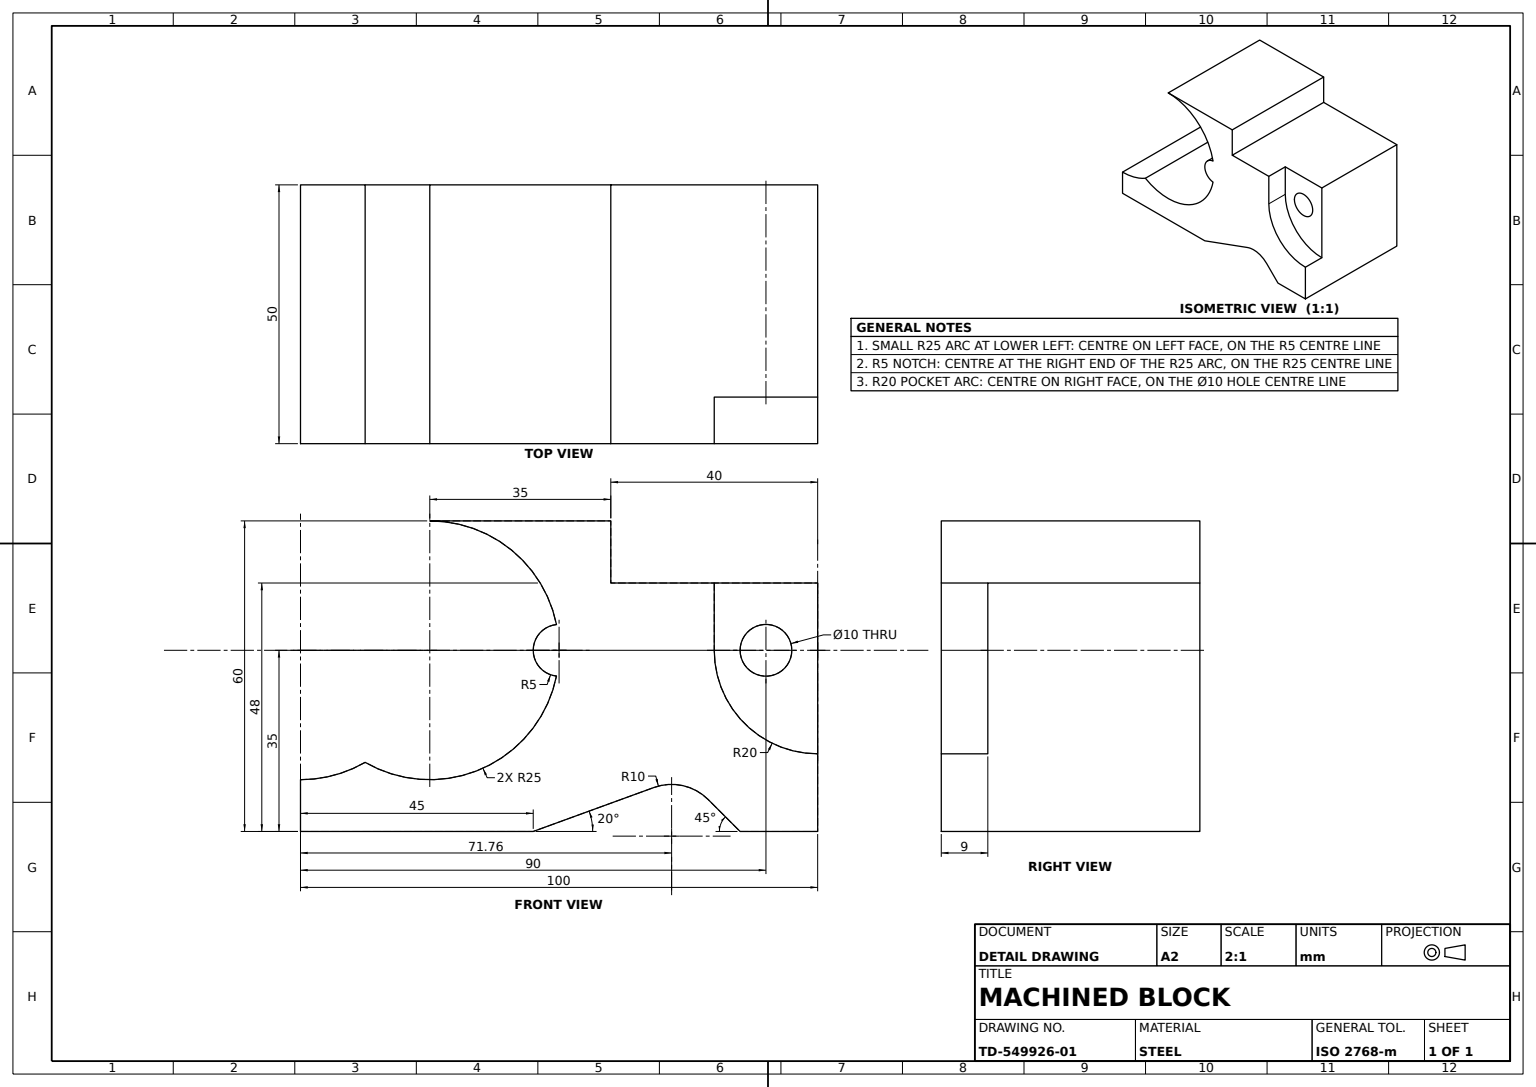
ISO-10303-21;
HEADER;
FILE_DESCRIPTION((''),'2;1');
FILE_NAME('','',(''),(''),'','','');
FILE_SCHEMA(('AUTOMOTIVE_DESIGN'));
ENDSEC;
DATA;
#1=APPLICATION_CONTEXT('');
#2=PRODUCT_CONTEXT('',#1,'mechanical');
#3=PRODUCT('','','',(#2));
#4=PRODUCT_DEFINITION_FORMATION('','',#3);
#5=PRODUCT_DEFINITION_CONTEXT('',#1,'design');
#6=PRODUCT_DEFINITION('','',#4,#5);
#7=PRODUCT_DEFINITION_SHAPE('','',#6);
#8=(LENGTH_UNIT()NAMED_UNIT(*)SI_UNIT(.MILLI.,.METRE.));
#9=(NAMED_UNIT(*)PLANE_ANGLE_UNIT()SI_UNIT($,.RADIAN.));
#10=(NAMED_UNIT(*)SI_UNIT($,.STERADIAN.)SOLID_ANGLE_UNIT());
#11=UNCERTAINTY_MEASURE_WITH_UNIT(LENGTH_MEASURE(1.E-05),#8,'distance_accuracy_value','');
#12=(GEOMETRIC_REPRESENTATION_CONTEXT(3)GLOBAL_UNCERTAINTY_ASSIGNED_CONTEXT((#11))GLOBAL_UNIT_ASSIGNED_CONTEXT((#8,#9,#10))REPRESENTATION_CONTEXT('',''));
#13=CARTESIAN_POINT('',(85.,35.,-25.));
#14=VERTEX_POINT('',#13);
#15=CARTESIAN_POINT('',(85.,35.,16.));
#16=VERTEX_POINT('',#15);
#17=CARTESIAN_POINT('',(85.,35.,-101.));
#18=DIRECTION('',(0.,0.,1.));
#19=VECTOR('',#18,1000.);
#20=LINE('',#17,#19);
#21=EDGE_CURVE('',#14,#16,#20,.T.);
#22=ORIENTED_EDGE('',*,*,#21,.F.);
#23=CARTESIAN_POINT('',(95.,35.,-25.));
#24=VERTEX_POINT('',#23);
#25=CARTESIAN_POINT('',(90.,35.,-25.));
#26=DIRECTION('',(1.,0.,0.));
#27=AXIS2_PLACEMENT_3D('',#25,#18,#26);
#28=CIRCLE('',#27,5.);
#29=EDGE_CURVE('',#24,#14,#28,.T.);
#30=ORIENTED_EDGE('',*,*,#29,.F.);
#31=CARTESIAN_POINT('',(95.,35.,16.));
#32=VERTEX_POINT('',#31);
#33=CARTESIAN_POINT('',(95.,35.,-101.));
#34=LINE('',#33,#19);
#35=EDGE_CURVE('',#24,#32,#34,.T.);
#36=ORIENTED_EDGE('',*,*,#35,.T.);
#37=CARTESIAN_POINT('',(90.,35.,16.));
#38=AXIS2_PLACEMENT_3D('',#37,#18,#26);
#39=CIRCLE('',#38,5.);
#40=EDGE_CURVE('',#32,#16,#39,.T.);
#41=ORIENTED_EDGE('',*,*,#40,.T.);
#42=EDGE_LOOP('',(#22,#30,#36,#41));
#43=FACE_OUTER_BOUND('',#42,.T.);
#44=CARTESIAN_POINT('',(90.,35.,-101.));
#45=AXIS2_PLACEMENT_3D('',#44,#18,#26);
#46=CYLINDRICAL_SURFACE('',#45,5.);
#47=ADVANCED_FACE('',(#43),#46,.F.);
#48=CARTESIAN_POINT('',(0.,0.,25.));
#49=VERTEX_POINT('',#48);
#50=CARTESIAN_POINT('',(0.,0.,-25.));
#51=VERTEX_POINT('',#50);
#52=DIRECTION('',(0.,0.,-1.));
#53=VECTOR('',#52,1000.);
#54=LINE('',#48,#53);
#55=EDGE_CURVE('',#49,#51,#54,.T.);
#56=ORIENTED_EDGE('',*,*,#55,.T.);
#57=CARTESIAN_POINT('',(45.,0.,-25.));
#58=VERTEX_POINT('',#57);
#59=VECTOR('',#26,1000.);
#60=LINE('',#50,#59);
#61=EDGE_CURVE('',#51,#58,#60,.T.);
#62=ORIENTED_EDGE('',*,*,#61,.T.);
#63=CARTESIAN_POINT('',(45.,0.,25.));
#64=VERTEX_POINT('',#63);
#65=LINE('',#57,#19);
#66=EDGE_CURVE('',#58,#64,#65,.T.);
#67=ORIENTED_EDGE('',*,*,#66,.T.);
#68=LINE('',#48,#59);
#69=EDGE_CURVE('',#49,#64,#68,.T.);
#70=ORIENTED_EDGE('',*,*,#69,.F.);
#71=EDGE_LOOP('',(#56,#62,#67,#70));
#72=FACE_OUTER_BOUND('',#71,.T.);
#73=DIRECTION('',(0.,1.,0.));
#74=AXIS2_PLACEMENT_3D('',#48,#73,#18);
#75=PLANE('',#74);
#76=ADVANCED_FACE('',(#72),#75,.F.);
#77=CARTESIAN_POINT('',(25.,60.,25.));
#78=VERTEX_POINT('',#77);
#79=CARTESIAN_POINT('',(25.,60.,-25.));
#80=VERTEX_POINT('',#79);
#81=LINE('',#77,#53);
#82=EDGE_CURVE('',#78,#80,#81,.T.);
#83=ORIENTED_EDGE('',*,*,#82,.F.);
#84=CARTESIAN_POINT('',(60.,60.,25.));
#85=VERTEX_POINT('',#84);
#86=CARTESIAN_POINT('',(0.,60.,25.));
#87=LINE('',#86,#59);
#88=EDGE_CURVE('',#78,#85,#87,.T.);
#89=ORIENTED_EDGE('',*,*,#88,.T.);
#90=CARTESIAN_POINT('',(60.,60.,-25.));
#91=VERTEX_POINT('',#90);
#92=LINE('',#84,#53);
#93=EDGE_CURVE('',#85,#91,#92,.T.);
#94=ORIENTED_EDGE('',*,*,#93,.T.);
#95=CARTESIAN_POINT('',(0.,60.,-25.));
#96=LINE('',#95,#59);
#97=EDGE_CURVE('',#80,#91,#96,.T.);
#98=ORIENTED_EDGE('',*,*,#97,.F.);
#99=EDGE_LOOP('',(#83,#89,#94,#98));
#100=FACE_OUTER_BOUND('',#99,.T.);
#101=AXIS2_PLACEMENT_3D('',#86,#73,#18);
#102=PLANE('',#101);
#103=ADVANCED_FACE('',(#100),#102,.T.);
#104=CARTESIAN_POINT('',(0.,10.,25.));
#105=VERTEX_POINT('',#104);
#106=CARTESIAN_POINT('',(0.,10.,-25.));
#107=VERTEX_POINT('',#106);
#108=LINE('',#104,#53);
#109=EDGE_CURVE('',#105,#107,#108,.T.);
#110=ORIENTED_EDGE('',*,*,#109,.F.);
#111=CARTESIAN_POINT('',(12.5,13.349365,25.));
#112=VERTEX_POINT('',#111);
#113=CARTESIAN_POINT('',(0.,35.,25.));
#114=AXIS2_PLACEMENT_3D('',#113,#18,#26);
#115=CIRCLE('',#114,25.);
#116=EDGE_CURVE('',#105,#112,#115,.T.);
#117=ORIENTED_EDGE('',*,*,#116,.T.);
#118=CARTESIAN_POINT('',(12.5,13.349365,-25.));
#119=VERTEX_POINT('',#118);
#120=CARTESIAN_POINT('',(12.5,13.349365,0.));
#121=LINE('',#120,#19);
#122=EDGE_CURVE('',#119,#112,#121,.T.);
#123=ORIENTED_EDGE('',*,*,#122,.F.);
#124=CARTESIAN_POINT('',(0.,35.,-25.));
#125=AXIS2_PLACEMENT_3D('',#124,#18,#26);
#126=CIRCLE('',#125,25.);
#127=EDGE_CURVE('',#107,#119,#126,.T.);
#128=ORIENTED_EDGE('',*,*,#127,.F.);
#129=EDGE_LOOP('',(#110,#117,#123,#128));
#130=FACE_OUTER_BOUND('',#129,.T.);
#131=DIRECTION('',(-1.,0.,0.));
#132=AXIS2_PLACEMENT_3D('',#113,#52,#131);
#133=CYLINDRICAL_SURFACE('',#132,25.);
#134=ADVANCED_FACE('',(#130),#133,.F.);
#135=CARTESIAN_POINT('',(85.,0.,-25.));
#136=VERTEX_POINT('',#135);
#137=CARTESIAN_POINT('',(85.,0.,25.));
#138=VERTEX_POINT('',#137);
#139=LINE('',#135,#19);
#140=EDGE_CURVE('',#136,#138,#139,.T.);
#141=ORIENTED_EDGE('',*,*,#140,.F.);
#142=CARTESIAN_POINT('',(100.,0.,-25.));
#143=VERTEX_POINT('',#142);
#144=EDGE_CURVE('',#136,#143,#60,.T.);
#145=ORIENTED_EDGE('',*,*,#144,.T.);
#146=CARTESIAN_POINT('',(100.,0.,25.));
#147=VERTEX_POINT('',#146);
#148=LINE('',#146,#53);
#149=EDGE_CURVE('',#147,#143,#148,.T.);
#150=ORIENTED_EDGE('',*,*,#149,.F.);
#151=EDGE_CURVE('',#138,#147,#68,.T.);
#152=ORIENTED_EDGE('',*,*,#151,.F.);
#153=EDGE_LOOP('',(#141,#145,#150,#152));
#154=FACE_OUTER_BOUND('',#153,.T.);
#155=ADVANCED_FACE('',(#154),#75,.F.);
#156=CARTESIAN_POINT('',(78.83092,6.16908,-25.));
#157=VERTEX_POINT('',#156);
#158=CARTESIAN_POINT('',(68.339651,8.494938,-25.));
#159=VERTEX_POINT('',#158);
#160=CARTESIAN_POINT('',(71.759852,-0.901988,-25.));
#161=AXIS2_PLACEMENT_3D('',#160,#18,#131);
#162=CIRCLE('',#161,10.);
#163=EDGE_CURVE('',#157,#159,#162,.T.);
#164=ORIENTED_EDGE('',*,*,#163,.F.);
#165=CARTESIAN_POINT('',(78.83092,6.16908,25.));
#166=VERTEX_POINT('',#165);
#167=LINE('',#156,#19);
#168=EDGE_CURVE('',#157,#166,#167,.T.);
#169=ORIENTED_EDGE('',*,*,#168,.T.);
#170=CARTESIAN_POINT('',(68.339651,8.494938,25.));
#171=VERTEX_POINT('',#170);
#172=CARTESIAN_POINT('',(71.759852,-0.901988,25.));
#173=AXIS2_PLACEMENT_3D('',#172,#18,#131);
#174=CIRCLE('',#173,10.);
#175=EDGE_CURVE('',#166,#171,#174,.T.);
#176=ORIENTED_EDGE('',*,*,#175,.T.);
#177=LINE('',#158,#19);
#178=EDGE_CURVE('',#159,#171,#177,.T.);
#179=ORIENTED_EDGE('',*,*,#178,.F.);
#180=EDGE_LOOP('',(#164,#169,#176,#179));
#181=FACE_OUTER_BOUND('',#180,.T.);
#182=AXIS2_PLACEMENT_3D('',#160,#18,#26);
#183=CYLINDRICAL_SURFACE('',#182,10.);
#184=ADVANCED_FACE('',(#181),#183,.F.);
#185=CARTESIAN_POINT('',(49.5,39.974937,25.));
#186=VERTEX_POINT('',#185);
#187=CARTESIAN_POINT('',(25.,35.,25.));
#188=AXIS2_PLACEMENT_3D('',#187,#18,#26);
#189=CIRCLE('',#188,25.);
#190=EDGE_CURVE('',#186,#78,#189,.T.);
#191=ORIENTED_EDGE('',*,*,#190,.F.);
#192=CARTESIAN_POINT('',(49.5,30.025063,25.));
#193=VERTEX_POINT('',#192);
#194=CARTESIAN_POINT('',(50.,35.,25.));
#195=AXIS2_PLACEMENT_3D('',#194,#18,#26);
#196=CIRCLE('',#195,5.);
#197=EDGE_CURVE('',#186,#193,#196,.T.);
#198=ORIENTED_EDGE('',*,*,#197,.T.);
#199=EDGE_CURVE('',#112,#193,#189,.T.);
#200=ORIENTED_EDGE('',*,*,#199,.F.);
#201=ORIENTED_EDGE('',*,*,#116,.F.);
#202=VECTOR('',#73,1000.);
#203=LINE('',#48,#202);
#204=EDGE_CURVE('',#49,#105,#203,.T.);
#205=ORIENTED_EDGE('',*,*,#204,.F.);
#206=ORIENTED_EDGE('',*,*,#69,.T.);
#207=DIRECTION('',(-0.939692621,-0.342020143,0.));
#208=VECTOR('',#207,1000.);
#209=LINE('',#63,#208);
#210=EDGE_CURVE('',#171,#64,#209,.T.);
#211=ORIENTED_EDGE('',*,*,#210,.F.);
#212=ORIENTED_EDGE('',*,*,#175,.F.);
#213=DIRECTION('',(-0.707106781,0.707106781,0.));
#214=VECTOR('',#213,1000.);
#215=LINE('',#137,#214);
#216=EDGE_CURVE('',#138,#166,#215,.T.);
#217=ORIENTED_EDGE('',*,*,#216,.F.);
#218=ORIENTED_EDGE('',*,*,#151,.T.);
#219=CARTESIAN_POINT('',(100.,15.,25.));
#220=VERTEX_POINT('',#219);
#221=LINE('',#146,#202);
#222=EDGE_CURVE('',#147,#220,#221,.T.);
#223=ORIENTED_EDGE('',*,*,#222,.T.);
#224=CARTESIAN_POINT('',(80.,35.,25.));
#225=VERTEX_POINT('',#224);
#226=CARTESIAN_POINT('',(100.,35.,25.));
#227=AXIS2_PLACEMENT_3D('',#226,#18,#26);
#228=CIRCLE('',#227,20.);
#229=EDGE_CURVE('',#225,#220,#228,.T.);
#230=ORIENTED_EDGE('',*,*,#229,.F.);
#231=CARTESIAN_POINT('',(80.,48.,25.));
#232=VERTEX_POINT('',#231);
#233=DIRECTION('',(0.,-1.,0.));
#234=VECTOR('',#233,1000.);
#235=LINE('',#224,#234);
#236=EDGE_CURVE('',#232,#225,#235,.T.);
#237=ORIENTED_EDGE('',*,*,#236,.F.);
#238=CARTESIAN_POINT('',(60.,48.,25.));
#239=VERTEX_POINT('',#238);
#240=CARTESIAN_POINT('',(0.,48.,25.));
#241=VECTOR('',#131,1000.);
#242=LINE('',#240,#241);
#243=EDGE_CURVE('',#232,#239,#242,.T.);
#244=ORIENTED_EDGE('',*,*,#243,.T.);
#245=CARTESIAN_POINT('',(60.,0.,25.));
#246=LINE('',#245,#202);
#247=EDGE_CURVE('',#239,#85,#246,.T.);
#248=ORIENTED_EDGE('',*,*,#247,.T.);
#249=ORIENTED_EDGE('',*,*,#88,.F.);
#250=EDGE_LOOP('',(#191,#198,#200,#201,#205,#206,#211,#212,#217,#218,#223,#230,#237,#244,#248,#249));
#251=FACE_OUTER_BOUND('',#250,.T.);
#252=AXIS2_PLACEMENT_3D('',#48,#18,#26);
#253=PLANE('',#252);
#254=ADVANCED_FACE('',(#251),#253,.T.);
#255=CARTESIAN_POINT('',(100.,48.,-25.));
#256=VERTEX_POINT('',#255);
#257=CARTESIAN_POINT('',(60.,48.,-25.));
#258=VERTEX_POINT('',#257);
#259=CARTESIAN_POINT('',(0.,48.,-25.));
#260=LINE('',#259,#241);
#261=EDGE_CURVE('',#256,#258,#260,.T.);
#262=ORIENTED_EDGE('',*,*,#261,.T.);
#263=LINE('',#238,#53);
#264=EDGE_CURVE('',#239,#258,#263,.T.);
#265=ORIENTED_EDGE('',*,*,#264,.F.);
#266=ORIENTED_EDGE('',*,*,#243,.F.);
#267=CARTESIAN_POINT('',(80.,48.,16.));
#268=VERTEX_POINT('',#267);
#269=LINE('',#267,#19);
#270=EDGE_CURVE('',#268,#232,#269,.T.);
#271=ORIENTED_EDGE('',*,*,#270,.F.);
#272=CARTESIAN_POINT('',(100.,48.,16.));
#273=VERTEX_POINT('',#272);
#274=LINE('',#267,#241);
#275=EDGE_CURVE('',#273,#268,#274,.T.);
#276=ORIENTED_EDGE('',*,*,#275,.F.);
#277=CARTESIAN_POINT('',(100.,48.,25.));
#278=LINE('',#277,#53);
#279=EDGE_CURVE('',#273,#256,#278,.T.);
#280=ORIENTED_EDGE('',*,*,#279,.T.);
#281=EDGE_LOOP('',(#262,#265,#266,#271,#276,#280));
#282=FACE_OUTER_BOUND('',#281,.T.);
#283=AXIS2_PLACEMENT_3D('',#240,#233,#52);
#284=PLANE('',#283);
#285=ADVANCED_FACE('',(#282),#284,.F.);
#286=ORIENTED_EDGE('',*,*,#199,.T.);
#287=CARTESIAN_POINT('',(49.5,30.025063,-25.));
#288=VERTEX_POINT('',#287);
#289=CARTESIAN_POINT('',(49.5,30.025063,0.));
#290=LINE('',#289,#53);
#291=EDGE_CURVE('',#193,#288,#290,.T.);
#292=ORIENTED_EDGE('',*,*,#291,.T.);
#293=CARTESIAN_POINT('',(25.,35.,-25.));
#294=AXIS2_PLACEMENT_3D('',#293,#18,#26);
#295=CIRCLE('',#294,25.);
#296=EDGE_CURVE('',#119,#288,#295,.T.);
#297=ORIENTED_EDGE('',*,*,#296,.F.);
#298=ORIENTED_EDGE('',*,*,#122,.T.);
#299=EDGE_LOOP('',(#286,#292,#297,#298));
#300=FACE_OUTER_BOUND('',#299,.T.);
#301=CYLINDRICAL_SURFACE('',#294,25.);
#302=ADVANCED_FACE('',(#300),#301,.F.);
#303=EDGE_CURVE('',#14,#24,#28,.T.);
#304=ORIENTED_EDGE('',*,*,#303,.F.);
#305=ORIENTED_EDGE('',*,*,#21,.T.);
#306=EDGE_CURVE('',#16,#32,#39,.T.);
#307=ORIENTED_EDGE('',*,*,#306,.T.);
#308=ORIENTED_EDGE('',*,*,#35,.F.);
#309=EDGE_LOOP('',(#304,#305,#307,#308));
#310=FACE_OUTER_BOUND('',#309,.T.);
#311=ADVANCED_FACE('',(#310),#46,.F.);
#312=ORIENTED_EDGE('',*,*,#291,.F.);
#313=ORIENTED_EDGE('',*,*,#197,.F.);
#314=CARTESIAN_POINT('',(49.5,39.974937,-25.));
#315=VERTEX_POINT('',#314);
#316=CARTESIAN_POINT('',(49.5,39.974937,0.));
#317=LINE('',#316,#19);
#318=EDGE_CURVE('',#315,#186,#317,.T.);
#319=ORIENTED_EDGE('',*,*,#318,.F.);
#320=CARTESIAN_POINT('',(50.,35.,-25.));
#321=AXIS2_PLACEMENT_3D('',#320,#18,#26);
#322=CIRCLE('',#321,5.);
#323=EDGE_CURVE('',#315,#288,#322,.T.);
#324=ORIENTED_EDGE('',*,*,#323,.T.);
#325=EDGE_LOOP('',(#312,#313,#319,#324));
#326=FACE_OUTER_BOUND('',#325,.T.);
#327=CYLINDRICAL_SURFACE('',#321,5.);
#328=ADVANCED_FACE('',(#326),#327,.T.);
#329=ORIENTED_EDGE('',*,*,#204,.T.);
#330=ORIENTED_EDGE('',*,*,#109,.T.);
#331=LINE('',#50,#202);
#332=EDGE_CURVE('',#51,#107,#331,.T.);
#333=ORIENTED_EDGE('',*,*,#332,.F.);
#334=ORIENTED_EDGE('',*,*,#55,.F.);
#335=EDGE_LOOP('',(#329,#330,#333,#334));
#336=FACE_OUTER_BOUND('',#335,.T.);
#337=AXIS2_PLACEMENT_3D('',#48,#131,#18);
#338=PLANE('',#337);
#339=ADVANCED_FACE('',(#336),#338,.T.);
#340=ORIENTED_EDGE('',*,*,#190,.T.);
#341=ORIENTED_EDGE('',*,*,#82,.T.);
#342=EDGE_CURVE('',#315,#80,#295,.T.);
#343=ORIENTED_EDGE('',*,*,#342,.F.);
#344=ORIENTED_EDGE('',*,*,#318,.T.);
#345=EDGE_LOOP('',(#340,#341,#343,#344));
#346=FACE_OUTER_BOUND('',#345,.T.);
#347=ADVANCED_FACE('',(#346),#301,.F.);
#348=ORIENTED_EDGE('',*,*,#247,.F.);
#349=ORIENTED_EDGE('',*,*,#264,.T.);
#350=CARTESIAN_POINT('',(60.,0.,-25.));
#351=LINE('',#350,#202);
#352=EDGE_CURVE('',#258,#91,#351,.T.);
#353=ORIENTED_EDGE('',*,*,#352,.T.);
#354=ORIENTED_EDGE('',*,*,#93,.F.);
#355=EDGE_LOOP('',(#348,#349,#353,#354));
#356=FACE_OUTER_BOUND('',#355,.T.);
#357=AXIS2_PLACEMENT_3D('',#245,#131,#18);
#358=PLANE('',#357);
#359=ADVANCED_FACE('',(#356),#358,.F.);
#360=ORIENTED_EDGE('',*,*,#261,.F.);
#361=LINE('',#142,#202);
#362=EDGE_CURVE('',#143,#256,#361,.T.);
#363=ORIENTED_EDGE('',*,*,#362,.F.);
#364=ORIENTED_EDGE('',*,*,#144,.F.);
#365=LINE('',#135,#214);
#366=EDGE_CURVE('',#136,#157,#365,.T.);
#367=ORIENTED_EDGE('',*,*,#366,.T.);
#368=ORIENTED_EDGE('',*,*,#163,.T.);
#369=LINE('',#57,#208);
#370=EDGE_CURVE('',#159,#58,#369,.T.);
#371=ORIENTED_EDGE('',*,*,#370,.T.);
#372=ORIENTED_EDGE('',*,*,#61,.F.);
#373=ORIENTED_EDGE('',*,*,#332,.T.);
#374=ORIENTED_EDGE('',*,*,#127,.T.);
#375=ORIENTED_EDGE('',*,*,#296,.T.);
#376=ORIENTED_EDGE('',*,*,#323,.F.);
#377=ORIENTED_EDGE('',*,*,#342,.T.);
#378=ORIENTED_EDGE('',*,*,#97,.T.);
#379=ORIENTED_EDGE('',*,*,#352,.F.);
#380=EDGE_LOOP('',(#360,#363,#364,#367,#368,#371,#372,#373,#374,#375,#376,#377,#378,#379));
#381=FACE_OUTER_BOUND('',#380,.T.);
#382=ORIENTED_EDGE('',*,*,#303,.T.);
#383=ORIENTED_EDGE('',*,*,#29,.T.);
#384=EDGE_LOOP('',(#382,#383));
#385=FACE_BOUND('',#384,.T.);
#386=AXIS2_PLACEMENT_3D('',#50,#18,#26);
#387=PLANE('',#386);
#388=ADVANCED_FACE('',(#381,#385),#387,.F.);
#389=ORIENTED_EDGE('',*,*,#366,.F.);
#390=ORIENTED_EDGE('',*,*,#140,.T.);
#391=ORIENTED_EDGE('',*,*,#216,.T.);
#392=ORIENTED_EDGE('',*,*,#168,.F.);
#393=EDGE_LOOP('',(#389,#390,#391,#392));
#394=FACE_OUTER_BOUND('',#393,.T.);
#395=DIRECTION('',(0.707106781,0.707106781,0.));
#396=AXIS2_PLACEMENT_3D('',#135,#395,#213);
#397=PLANE('',#396);
#398=ADVANCED_FACE('',(#394),#397,.F.);
#399=ORIENTED_EDGE('',*,*,#279,.F.);
#400=CARTESIAN_POINT('',(100.,15.,16.));
#401=VERTEX_POINT('',#400);
#402=LINE('',#272,#202);
#403=EDGE_CURVE('',#401,#273,#402,.T.);
#404=ORIENTED_EDGE('',*,*,#403,.F.);
#405=LINE('',#400,#19);
#406=EDGE_CURVE('',#401,#220,#405,.T.);
#407=ORIENTED_EDGE('',*,*,#406,.T.);
#408=ORIENTED_EDGE('',*,*,#222,.F.);
#409=ORIENTED_EDGE('',*,*,#149,.T.);
#410=ORIENTED_EDGE('',*,*,#362,.T.);
#411=EDGE_LOOP('',(#399,#404,#407,#408,#409,#410));
#412=FACE_OUTER_BOUND('',#411,.T.);
#413=AXIS2_PLACEMENT_3D('',#146,#131,#18);
#414=PLANE('',#413);
#415=ADVANCED_FACE('',(#412),#414,.F.);
#416=ORIENTED_EDGE('',*,*,#370,.F.);
#417=ORIENTED_EDGE('',*,*,#178,.T.);
#418=ORIENTED_EDGE('',*,*,#210,.T.);
#419=ORIENTED_EDGE('',*,*,#66,.F.);
#420=EDGE_LOOP('',(#416,#417,#418,#419));
#421=FACE_OUTER_BOUND('',#420,.T.);
#422=DIRECTION('',(-0.342020143,0.939692621,0.));
#423=AXIS2_PLACEMENT_3D('',#57,#422,#207);
#424=PLANE('',#423);
#425=ADVANCED_FACE('',(#421),#424,.F.);
#426=ORIENTED_EDGE('',*,*,#270,.T.);
#427=ORIENTED_EDGE('',*,*,#236,.T.);
#428=CARTESIAN_POINT('',(80.,35.,16.));
#429=VERTEX_POINT('',#428);
#430=LINE('',#428,#19);
#431=EDGE_CURVE('',#429,#225,#430,.T.);
#432=ORIENTED_EDGE('',*,*,#431,.F.);
#433=LINE('',#428,#234);
#434=EDGE_CURVE('',#268,#429,#433,.T.);
#435=ORIENTED_EDGE('',*,*,#434,.F.);
#436=EDGE_LOOP('',(#426,#427,#432,#435));
#437=FACE_OUTER_BOUND('',#436,.T.);
#438=AXIS2_PLACEMENT_3D('',#428,#131,#18);
#439=PLANE('',#438);
#440=ADVANCED_FACE('',(#437),#439,.F.);
#441=ORIENTED_EDGE('',*,*,#431,.T.);
#442=ORIENTED_EDGE('',*,*,#229,.T.);
#443=ORIENTED_EDGE('',*,*,#406,.F.);
#444=CARTESIAN_POINT('',(100.,35.,16.));
#445=AXIS2_PLACEMENT_3D('',#444,#18,#26);
#446=CIRCLE('',#445,20.);
#447=EDGE_CURVE('',#429,#401,#446,.T.);
#448=ORIENTED_EDGE('',*,*,#447,.F.);
#449=EDGE_LOOP('',(#441,#442,#443,#448));
#450=FACE_OUTER_BOUND('',#449,.T.);
#451=CYLINDRICAL_SURFACE('',#445,20.);
#452=ADVANCED_FACE('',(#450),#451,.F.);
#453=ORIENTED_EDGE('',*,*,#40,.F.);
#454=ORIENTED_EDGE('',*,*,#306,.F.);
#455=EDGE_LOOP('',(#453,#454));
#456=FACE_BOUND('',#455,.T.);
#457=ORIENTED_EDGE('',*,*,#275,.T.);
#458=ORIENTED_EDGE('',*,*,#434,.T.);
#459=ORIENTED_EDGE('',*,*,#447,.T.);
#460=ORIENTED_EDGE('',*,*,#403,.T.);
#461=EDGE_LOOP('',(#457,#458,#459,#460));
#462=FACE_OUTER_BOUND('',#461,.T.);
#463=PLANE('',#445);
#464=ADVANCED_FACE('',(#456,#462),#463,.T.);
#465=CLOSED_SHELL('',(#47,#76,#103,#134,#155,#184,#254,#285,#302,#311,#328,#339,#347,#359,#388,#398,#415,#425,#440,#452,#464));
#466=MANIFOLD_SOLID_BREP('',#465);
#467=ADVANCED_BREP_SHAPE_REPRESENTATION('',(#466),#12);
#468=SHAPE_DEFINITION_REPRESENTATION(#7,#467);
ENDSEC;
END-ISO-10303-21;
